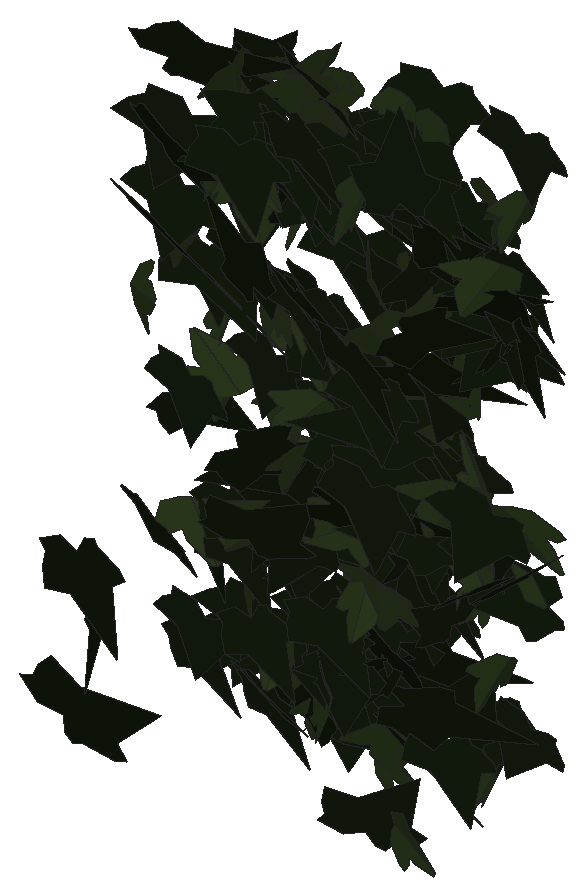
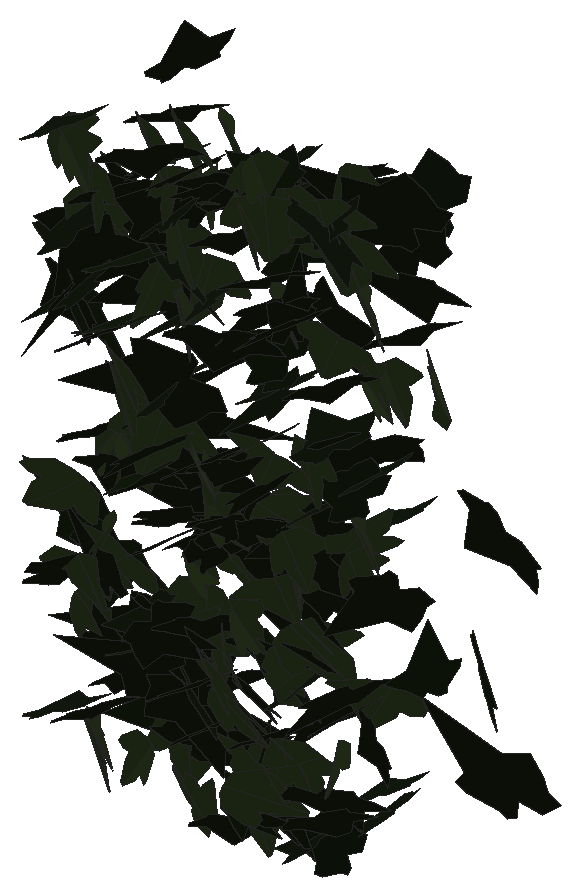
# SketchUp Ruby script. Lengths in millimetres.
U = 1.mm
M = Sketchup.active_model
def pt(a) = Geom::Point3d.new(a.map { |v| v * U })
def face(e, loops, mat)
  f = e.add_face(loops[0].map { |a| pt(a) })
  loops[1..].each { |l| e.add_face(l.map { |a| pt(a) }).erase! }
  f.material = f.back_material = mat if mat
  f
end
# faces: each face lists its corners as indices into pts; further lists are holes
def faces(e, pts, list, mat = nil) = list.each { |f| face(e, (f[0].is_a?(Array) ? f : [f]).map { |l| l.map { |i| pts[i] } }, mat) }
# xy, xz, yz: faces in a plane at the given z, y or x. An outline is a flat list of corners, or four numbers for a rectangle; further outlines are holes
def ring(l) = l.size == 4 ? [[l[0], l[1]], [l[2], l[1]], [l[2], l[3]], [l[0], l[3]]] : l.each_slice(2).to_a
def flat(e, list, mat, &to3) = list.each { |f| face(e, (f[0].is_a?(Array) ? f : [f]).map { |l| ring(l).map { |u, v| to3.(u, v) } }, mat) }
def xy(e, z, list, mat = nil) = flat(e, list, mat) { |x, y| [x, y, z] }
def xz(e, y, list, mat = nil) = flat(e, list, mat) { |x, z| [x, y, z] }
def yz(e, x, list, mat = nil) = flat(e, list, mat) { |y, z| [x, y, z] }
def lines(e, pts, list) = list.each { |a, b| e.add_line(pt(pts[a]), pt(pts[b])) }
# prism: a flat outline (further loops are holes) pulled along v
def prism(e, loops, v, mat = nil)
  f = face(e, loops, mat); d = Geom::Vector3d.new(v.map { |x| x * U })
  f.pushpull(f.normal.samedirection?(d) ? d.length : -d.length)
end
def box(e, o, s, mat = nil) = prism(e, [[o, [o[0] + s[0], o[1], o[2]], [o[0] + s[0], o[1] + s[1], o[2]], [o[0], o[1] + s[1], o[2]]]], [0, 0, s[2]], mat)
def at(x, y, z, deg = 0) = Geom::Transformation.translation(pt([x, y, z])) * Geom::Transformation.rotation(ORIGIN, Z_AXIS, deg.degrees)
def axes(o, x, y, z) = Geom::Transformation.new([*x, 0, *y, 0, *z, 0, *pt(o).to_a, 1])
def part(name) = M.definitions.add(name)
# library, detail: a bought-in or finely detailed component or shape, given as its bounding box
def library(name, o, s) = part(name).tap { |d| box(d.entities, o, s) }
def detail(e, o, s) = box(e.add_group.entities, o, s)
def put(e, d, t, mat = nil) = e.add_instance(d, t).tap { |i| i.material = mat if mat }
def group(e, t, mat = nil) = e.add_group.tap { |g| g.transformation = t; g.material = mat if mat }.entities
root = M.entities
M.materials.add("efeu1").color = [18, 25, 13]
M.materials.add("efeu2").color = [43, 57, 29]
c1 = part("ivyleaf_9")
p = [[39.1,54.8,31.7],[34.5,51.8,30.2],[-5.3,25.2,17.3],[-17.9,28.3,20.9],[-21.6,21.7,17],[-20.2,4.3,5.3],
  [-22.9,-0.3,2.5],[-17.1,-4,-0.6],[-2,-2.1,-1.2],[-0.7,-15.4,-10.1],[16.6,-22.3,-16.7],[21.1,-15.1,-12.5],
  [32.7,-10.7,-11],[46.1,-1.8,-6.6],[30.8,11.2,3.8]]
faces(c1.entities,p,[[0,1,2,3,4,5,6,7,8,9,10,11,12,13,14]],"efeu1")
c2 = part("ivyleaf_10")
p = [[0,12.8,-0.8],[-1.5,51.3,-10.9],[-4.9,51,-11.6],[-13.6,26.5,-7.3],[-13.2,15.9,-4.6],[-21.1,19.3,-7.2],
  [-29.5,16.3,-8.3],[-29.2,8.3,-6.2],[-19.7,-9.8,0.5],[-7.6,-13,4],[1,-12.2,5.8],[-0.4,51.1,-11.1],
  [-1.5,51.1,-10.9],[1,-12.4,5.9],[16.9,-12.4,3.5],[35.1,9.1,-5.1],[35,12.9,-6.1],[20.5,16.4,-4.9],
  [15.8,15,-3.8],[15.3,27.6,-7.1],[12.8,31.3,-7.8]]
faces(c2.entities,p,[[0,1,2,3,4,5,6,7,8,9,10],[11,12,0,13,14,15,16,17,18,19,20]],"efeu2")
put(root,c1,axes([4063.2,733.8,2968.8],[-0.0376,-0.17228,-1.13576],[-0.13622,1.13391,-0.17075],[2.18206,0.06782,-0.03023]))
put(root,c1,axes([4055.8,686.5,2823.3],[1.5513,-0.70151,-0.67063],[0.96409,-0.43949,1.07541],[-1.57548,-0.95968,-0.00226]))
put(root,c1,axes([4064.7,770.6,3133.3],[-0.07341,-1.05593,0.33534],[0.00836,-0.33568,-1.05651],[2.10853,-0.03543,0.01586]))
put(root,c1,axes([4039.1,548.3,2628],[-0.17639,0.13273,1.43159],[1.7479,-1.09826,0.16129],[2.10526,0.92296,-0.01396]))
put(root,c2,axes([4084,770.9,3056],[1.04005,-0.97402,0.24753],[0.21534,-0.22034,-1.11681],[1.90052,0.55799,-0.00892]))
put(root,c1,axes([4066.9,765.7,2785.8],[-0.57531,0.08526,-1.02674],[1.87322,-0.29236,-0.31405],[-0.57954,-1.02961,0.00416]))
put(root,c1,axes([4093.4,699.6,3351.9],[-1.90869,-0.57528,-0.28926],[0.46815,0.15249,-1.15613],[1.13254,-1.03257,-0.00959]))
put(root,c1,axes([4080.8,559.1,2788],[-1.15251,0.38599,-1.26243],[2.05887,-0.65093,-0.71794],[-1.43996,-1.23965,-0.0161]))
put(root,c2,axes([4096.2,739.7,3231],[0.60383,-0.99417,0.40773],[0.17674,-0.39817,-1.04313],[2.03739,0.32919,-0.03035]))
put(root,c2,axes([4103.2,692.9,3216.8],[-0.05357,-1.12054,0.09049],[0.02713,-0.09087,-1.12077],[2.13938,-0.02691,0.01648]))
put(root,c2,axes([4080.5,728.4,2825.7],[1.80422,0.56567,0.28702],[0.45808,0.15674,-1.10388],[-1.11695,0.97801,0.01091]))
put(root,c1,axes([4097,683.1,3269.7],[-0.81375,-1.09553,0.2771],[-0.1636,-0.26388,-1.17591],[2.14444,-0.43585,0.01544]))
put(root,c1,axes([4079.5,718.6,2670],[0.7911,-1.03663,-0.23213],[-0.16867,0.21457,-1.11686],[2.01473,0.425,-0.00235]))
put(root,c2,axes([4080.7,628,3159],[0.3126,-0.42355,-1.17811],[0.73038,-1.11397,0.454],[-2.26797,-0.41712,-0.01618]))
put(root,c1,axes([4092.3,728.3,2690.3],[-0.54384,-0.962,0.52983],[0.06228,-0.55469,-0.98948],[2.08927,-0.23387,0.16741]))
put(root,c2,axes([4104,758.4,2997.4],[-0.27143,-1.03123,0.33808],[0.28146,-0.35627,-1.02434],[2.04614,-0.08779,0.18575]))
put(root,c1,axes([4089.7,744.9,3159.3],[-0.50804,-1.01056,-0.71541],[0.35516,0.69065,-1.04522],[2.32956,-0.32568,0.00333]))
put(root,c2,axes([4121.9,734.9,3008.2],[0.77762,1.07105,0.31506],[-0.32067,-0.27249,1.14486],[2.10045,-0.43812,0.05815]))
put(root,c1,axes([4080.9,770.3,3102.2],[0.96558,-0.86425,0.57784],[0.61724,-0.47932,-1.00165],[1.87988,0.60129,0.03208]))
put(root,c1,axes([4103.7,689.3,3023.2],[-0.28326,-1.04741,0.50626],[0.0019,-0.5105,-1.05589],[2.21408,-0.13356,0.06568]))
put(root,c2,axes([4132.2,737.6,3396.3],[-2.16895,-0.0376,0.07781],[-0.13713,-0.15481,-1.13008],[0.09082,-1.13175,0.15199]))
put(root,c1,axes([4075.9,695.7,3426.5],[0.48012,-0.09617,1.25178],[2.3233,-0.2795,-0.26749],[0.55821,1.24599,0.03662]))
put(root,c1,axes([4102.7,766.8,2838.7],[0.44567,-1.05433,-0.74965],[-0.12292,0.75136,-1.0769],[2.45905,0.22864,0.08203]))
put(root,c2,axes([4126.8,756.3,2744],[0.82972,-0.6078,-0.72659],[0.17893,0.82366,-0.63259],[1.79398,0.19896,0.39914]))
put(root,c1,axes([4137.5,778.4,2696.3],[-1.66468,-0.6183,-0.07224],[0.11368,0.04065,-1.07114],[1.17928,-0.87671,0.00128]))
put(root,c1,axes([4153.8,752.9,3420.1],[0.08478,0.9438,0.64907],[-0.50152,0.64059,-0.91338],[-2.12156,-0.11371,0.24185]))
put(root,c1,axes([4123.8,785.4,3238.9],[-0.65034,-1.10482,0.04804],[-0.04197,-0.04346,-1.15642],[2.10425,-0.34232,-0.00822]))
put(root,c1,axes([4136.9,786,2669],[-1.10183,-0.84086,0.1464],[-0.20736,-0.10265,-1.02041],[1.6111,-0.58827,-0.03121]))
put(root,c1,axes([4115.6,753.5,2798],[0.33532,-1.10949,-0.16604],[-0.05444,0.16358,-1.12339],[2.1344,0.17848,-0.00257]))
put(root,c2,axes([4137.4,699.6,3310],[0.97597,-1.06387,0.03588],[0.01726,-0.03545,-1.18099],[2.02583,0.51284,-0.00722]))
put(root,c1,axes([4107.7,638.6,3349.5],[0.086,-0.46985,1.26714],[0.91479,-1.17936,-0.45444],[2.4039,0.46561,0.1276]))
put(root,c2,axes([4147.8,726.4,3397.1],[0.79933,-1.10899,0.09128],[0.06289,-0.08509,-1.18585],[2.11683,0.42129,0.00077]))
put(root,c1,axes([4122.4,772,3153.9],[-0.13685,-1.03136,0.75937],[0.46641,-0.75759,-1.00574],[2.3925,0.0887,0.2395]))
put(root,c2,axes([4165.5,740.5,3428.7],[-1.23255,-0.9441,0.09396],[-0.11242,-0.07342,-1.14485],[1.80219,-0.65027,-0.00715]))
put(root,c1,axes([4120.9,756,2616.5],[0.97697,-0.63278,0.63099],[0.70112,-0.51313,-0.81428],[1.5495,0.63115,-0.0294]))
put(root,c1,axes([4126.4,458.7,2902.9],[-1.02872,-0.11963,-1.31812],[2.51895,-0.04442,-0.53871],[0.00785,-1.42395,0.12754]))
put(root,c2,axes([4166.7,683.2,3448.6],[-0.27581,-1.12045,-0.49738],[0.24984,0.48378,-1.12806],[2.31969,-0.18533,0.06236]))
put(root,c2,axes([4146.5,735.2,3264],[2.06754,-0.06274,0.33696],[0.64867,0.07925,-1.08406],[0.06902,1.13464,0.09435]))
put(root,c1,axes([4142.8,736.9,3426.8],[1.39004,-0.87128,-0.24651],[-0.13994,0.2586,-1.13184],[1.71762,0.72618,0.10729]))
put(root,c2,axes([4196.1,733.8,2858.6],[-1.04434,-0.88,0.71355],[-0.73332,-0.60063,-1.03704],[2.02769,-0.67046,-0.00754]))
put(root,c2,axes([4178,748.8,3115.7],[1.47628,-0.66922,-0.42703],[-0.16127,0.52383,-0.97484],[1.50225,0.71389,0.315]))
put(root,c1,axes([4168.2,759.3,3042.9],[-0.46422,-0.97099,0.50201],[-0.09726,-0.50367,-0.99902],[2.0781,-0.24048,0.06539]))
put(root,c2,axes([4190.4,768.4,2999.6],[-0.51307,-1.04797,0.25565],[0.04854,-0.26963,-1.07839],[2.05241,-0.2556,0.08941]))
put(root,c1,axes([4163.5,749.8,2617.7],[0.65941,-1.05732,0.04467],[0.02539,-0.04263,-1.11264],[2.01392,0.34673,-0.0006]))
put(root,c2,axes([4195,740.5,2691.7],[1.11846,0.84094,-0.38065],[-0.38381,-0.32338,-1.02576],[-1.71436,0.62103,-0.01869]))
put(root,c2,axes([4211.6,757.3,2808.7],[-0.53133,-0.24398,-1.07687],[-0.77106,-1.01065,0.33401],[-1.95487,0.46494,0.16095]))
put(root,c1,axes([4229.3,642.6,3213.2],[0.03014,-0.13978,1.28616],[-0.63687,1.24204,0.1391],[-2.37843,-0.33435,-0.02095]))
put(root,c1,axes([4179.6,772.6,3297.9],[0.58629,-1.0062,-0.49226],[0.01513,0.51248,-1.04257],[2.13183,0.27308,0.14278]))
put(root,c2,axes([4215.7,733.6,2967.4],[0.46874,-0.95429,-0.66969],[-0.25051,0.65733,-0.98509],[2.20461,0.27759,0.03045]))
put(root,c1,axes([4194.8,688.8,2740.6],[0.25993,-1.03082,-0.47157],[-0.1751,0.46334,-1.03946],[2.15028,0.16234,-0.02764]))
put(root,c1,axes([4194.1,747.9,2801.2],[0.26781,-1.01076,0.2547],[0.02641,-0.25517,-1.0203],[1.98364,0.13986,-0.0208]))
put(root,c2,axes([4213.9,761.5,2936.6],[1.33131,0.82364,-0.35405],[-0.50455,-0.23895,-1.07966],[-1.62994,0.74671,0.04503]))
put(root,c1,axes([4211.2,738.8,3263.6],[0.41262,0.63503,0.99661],[-1.08999,-0.82983,0.65335],[1.9673,-0.59297,0.15297]))
put(root,c1,axes([4219.6,720,2898.2],[-1.98469,0.24053,-0.72523],[1.35006,-0.15119,-1.07015],[-0.54036,-1.26118,-0.01002]))
put(root,c1,axes([4169.3,518.9,3338.8],[1.63551,-1.02214,0.66736],[0.7842,-0.52536,-1.33523],[2.18691,0.95281,-0.0203]))
put(root,c1,axes([4246.2,665.8,3407.3],[-2.01004,-0.45578,0.43483],[-0.76096,-0.17091,-1.15029],[0.92642,-1.12929,-0.00141]))
put(root,c1,axes([4256.3,714.5,2950.4],[0.02781,-0.01696,-1.27934],[-1.4668,-1.02137,0.00473],[-1.94369,0.77053,-0.02188]))
put(root,c1,axes([4200.7,663.2,2977],[0.17879,0.19429,-1.26731],[-0.15454,1.26906,0.18854],[2.43524,0.06627,0.10501]))
put(root,c2,axes([4227.6,767.2,3424.6],[-1.80513,-0.68999,0.0723],[0.0172,-0.13474,-1.16733],[1.32026,-0.94163,0.11406]))
put(root,c2,axes([4232.5,726.9,2696.3],[-1.66169,-0.55762,0.13382],[-0.19637,-0.08703,-1.03583],[1.07359,-0.879,0.01767]))
put(root,c2,axes([4230,737.8,3425],[-1.17,-0.98924,-0.02006],[0.02942,0.01401,-1.16468],[1.88288,-0.61492,0.00574]))
put(root,c2,axes([4243.1,789.2,2666.6],[-0.31222,-0.42953,1.0688],[-0.74455,-0.99464,-0.45977],[2.06195,-0.42419,-0.00418]))
put(root,c2,axes([4187.9,667.2,3353.5],[1.42353,-0.10302,0.86127],[1.62715,-0.1045,-0.75498],[0.2788,1.13593,0.00866]))
put(root,c1,axes([4261.4,719.4,2650.4],[0.19101,0.10696,-1.20825],[-2.29195,0.15384,-0.08641],[0.27619,1.20261,0.11852]))
put(root,c2,axes([4240.3,738.8,3012],[-0.67676,-0.66207,0.84033],[-0.21575,-0.85723,-0.72336],[2.0246,-0.31266,0.20381]))
put(root,c1,axes([4256.2,728.9,2830],[-1.01019,0.94881,-0.14514],[0.13472,-0.12671,-1.08718],[-1.8218,-0.53549,0.00009]))
put(root,c1,axes([4233.7,746.5,2842.2],[-1.52416,-0.56478,-0.39797],[0.63872,0.21455,-0.97982],[1.14939,-0.86815,0.01676]))
put(root,c1,axes([4218.6,776,3071.5],[0.26785,-1.08394,-0.35961],[-0.15113,0.35216,-1.09258],[2.16826,0.15845,-0.03173]))
put(root,c1,axes([4211.5,664.3,2865.5],[-0.91298,-0.1477,1.03329],[1.92257,-0.352,0.41866],[0.50015,1.08347,0.27687]))
put(root,c1,axes([4235.6,766.8,2730.8],[-0.81684,-0.85852,0.41648],[-0.21116,-0.40867,-0.95676],[1.80373,-0.43663,0.0766]))
put(root,c2,axes([4240.1,725.3,3280.5],[0.91907,-1.0045,0.19161],[0.15523,-0.17339,-1.11455],[1.94003,0.48974,-0.00159]))
put(root,c2,axes([4246.7,752.7,3461.9],[-0.17986,-1.17257,0.14511],[0.01943,-0.14638,-1.17617],[2.24857,-0.09253,0.02177]))
put(root,c1,axes([4222.1,743.5,3291.5],[0.40376,-0.83368,-0.79645],[-0.0522,0.80594,-0.85092],[2.19372,0.17262,0.12634]))
put(root,c1,axes([4225.7,777.1,3125],[0.01219,-1.15086,0.10669],[0.02355,-0.10662,-1.15082],[2.19959,0.00752,0.01173]))
put(root,c2,axes([4223.9,755.5,3093.8],[2.0494,-0.16577,0.40576],[0.76537,-0.05449,-1.08948],[0.33184,1.14944,0.00687]))
put(root,c1,axes([4253.4,714.1,2866.4],[-1.94468,0.00735,-0.47474],[0.90306,-0.02459,-1.02164],[-0.0324,-1.12643,0.01921]))
put(root,c1,axes([4227.1,730.5,3172.1],[1.47111,-0.68624,-0.53505],[-0.56535,0.46457,-1.02499],[1.55663,0.81727,0.13338]))
put(root,c2,axes([4255.7,755.3,2637.3],[-0.35167,-1.22293,0.12241],[-0.00071,-0.12373,-1.23668],[2.3391,-0.1839,0.01803]))
put(root,c1,axes([4235.2,613.4,3398.7],[-0.43152,-1.19319,-0.1831],[0.05445,0.18094,-1.21453],[2.29681,-0.22846,-0.00561]))
put(root,c2,axes([4256.8,772.2,3412.4],[1.0182,-1.03638,-0.20639],[-0.08709,0.2084,-1.16506],[2.00928,0.53421,0.05409]))
put(root,c2,axes([4258.3,771.3,2879.3],[0.16209,-1.01726,0.47014],[0.17797,-0.4634,-1.01962],[2.12538,0.11638,0.04952]))
put(root,c1,axes([4267.9,718.9,2704.5],[0.67268,-0.02431,-0.98557],[-1.57698,0.55999,-0.31097],[1.01667,0.88469,0.16975]))
put(root,c1,axes([4267.2,777.4,2652],[-0.98887,0.44648,-0.79608],[0.85806,-0.67094,-0.67055],[-1.51041,-0.67347,0.14026]))
put(root,c1,axes([4250.9,745.7,3315.9],[-0.77389,-1.0623,0.14187],[0.10768,-0.17281,-1.13176],[2.03687,-0.39447,0.11374]))
put(root,c1,axes([4241.9,724.3,3165.8],[-0.1396,-1.08728,0.2572],[0.21766,-0.26371,-1.08217],[2.11525,-0.04462,0.12833]))
put(root,c2,axes([4267,687.3,2987.1],[-0.11857,-1.19015,0.11543],[0.02693,-0.11631,-1.19161],[2.27556,-0.06064,0.02012]))
put(root,c1,axes([4235,739.7,3440.6],[0.46896,-0.86973,0.69875],[0.60117,-0.63192,-0.89794],[2.03643,0.38683,0.10417]))
put(root,c1,axes([4256.3,774.3,3007.7],[-0.9981,-0.92448,-0.39502],[0.43043,0.32563,-1.06233],[1.86431,-0.57012,0.03378]))
put(root,c1,axes([4259.1,780.5,2623.1],[-0.8878,-0.9233,-0.21395],[0.22109,0.18096,-1.03422],[1.79018,-0.48024,0.02163]))
put(root,c1,axes([4231.8,687.2,3323.5],[0.3995,-0.86177,0.88202],[0.82821,-0.78537,-0.87091],[2.19589,0.453,0.16801]))
put(root,c2,axes([4244.3,764,2689.7],[1.88644,-0.35344,0.57322],[1.01577,-0.20974,-1.0522],[0.7816,1.12564,-0.01607]))
put(root,c2,axes([4305.9,750.2,2748.5],[-0.42466,0.31031,0.98176],[-1.86084,0.25103,-0.30156],[-0.61425,-0.975,0.23482]))
put(root,c1,axes([4254.2,770.1,3008.1],[0.15289,-0.81349,-0.76492],[0.20511,0.76896,-0.80648],[2.11525,-0.01576,0.13349]))
put(root,c1,axes([4266.5,774,3382.7],[-0.6259,-1.10495,-0.04858],[0.02014,0.04754,-1.15284],[2.10487,-0.32902,-0.00342]))
put(root,c1,axes([4252.9,687.5,3401.1],[0.44117,-1.16401,0.1185],[0.05641,-0.11492,-1.18685],[2.22608,0.2336,0.00659]))
put(root,c2,axes([4291,694.2,2671.5],[0.82687,-0.91011,-0.76698],[-0.38138,0.74889,-1.00216],[2.23284,0.46495,0.11286]))
put(root,c2,axes([4279.5,714.5,3428.3],[-0.82873,-0.94744,-0.49277],[0.4694,0.42855,-1.04192],[1.97753,-0.49877,0.04081]))
put(root,c1,axes([4268.6,667.3,3393.4],[-0.17249,-1.14355,-0.11002],[-0.02181,0.11126,-1.14696],[2.18635,-0.08911,-0.02012]))
put(root,c1,axes([4268.9,765,3078],[-0.35831,-0.9964,-0.41796],[0.26952,0.39785,-1.01223],[2.0387,-0.22772,0.06036]))
put(root,c1,axes([4295.5,741.2,2780.2],[-1.77743,0.13526,-0.46488],[0.84083,-0.1751,-0.93849],[-0.37694,-1.02843,0.09865]))
put(root,c1,axes([4315.4,733.2,2752.8],[-1.60526,0.63927,-0.03384],[0.04785,-0.02285,-1.05833],[-1.21742,-0.84382,0.00302]))
put(root,c2,axes([4297,763,3002.7],[-0.05013,-0.95141,0.54361],[-0.02503,-0.54345,-0.95178],[2.0853,-0.02939,0.00164]))
put(root,c1,axes([4272.3,660.9,3419.6],[0.75304,-1.07385,-0.1602],[-0.04301,0.16232,-1.14391],[2.06593,0.3948,0.03458]))
put(root,c1,axes([4260.3,689.3,3185.6],[0.89518,-1.01293,0.6329],[0.52857,-0.56881,-1.11676],[2.21088,0.54612,0.01073]))
put(root,c2,axes([4300.4,776.3,2803.2],[1.34924,-0.7746,-0.0278],[-0.03338,0.02163,-1.05004],[1.4748,0.70915,0.00166]))
put(root,c1,axes([4294.3,766.8,3237.2],[-1.23484,-0.85152,-0.45532],[0.51845,0.36487,-1.07053],[1.7631,-0.70368,-0.00411]))
put(root,c2,axes([4286.4,762.3,2819],[0.84868,-0.5792,0.75887],[0.96948,-0.56401,-0.7298],[1.53662,0.67574,0.04132]))
put(root,c1,axes([4284.4,707.5,2774.5],[0.06898,-1.08694,-0.38663],[0.17408,0.38831,-1.08309],[2.18873,0.00337,0.09833]))
put(root,c2,axes([4325.1,700.7,2906.2],[1.57109,-0.44156,-0.64322],[-1.10336,0.27952,-0.93591],[0.99371,1.00849,-0.02223]))
put(root,c1,axes([4315,770.7,2943.2],[0.09758,0.06212,1.16836],[-1.35858,-0.92493,0.0805],[1.76429,-0.71568,-0.00263]))
put(root,c1,axes([4299.3,785,2984.3],[-0.16774,-1.09101,-0.08498],[0.02618,0.08414,-1.09454],[2.08253,-0.08894,0.00691]))
put(root,c2,axes([4294.6,790.6,3051.3],[-0.07594,-0.23287,-1.08262],[0.72149,-1.02074,0.20559],[-1.98022,-0.36297,0.11642]))
put(root,c1,axes([4308.4,711.5,2714.5],[-1.39712,-0.39739,-0.63975],[1.30419,0.01816,-0.7976],[0.59461,-0.97357,0.24625]))
put(root,c2,axes([4342.2,734.6,2814.5],[-1.8238,0.06982,0.44465],[-0.83984,0.06024,-0.96048],[-0.1687,-1.05469,-0.02542]))
put(root,c2,axes([4323.9,750.9,3028.6],[-0.42262,0.56884,-0.97487],[-0.09959,-0.99768,-0.57023],[-2.14582,-0.06573,0.21847]))
put(root,c1,axes([4317.9,768.1,2855],[-0.55826,-1.01734,-0.37749],[0.21614,0.36011,-1.05875],[2.05385,-0.31442,0.00881]))
put(root,c1,axes([4317.8,763.5,3063.1],[-0.22688,-1.19443,0.09383],[0.00222,-0.09441,-1.20032],[2.28025,-0.11875,0.0105]))
put(root,c1,axes([4373.3,711.5,2649],[-0.08153,0.23918,1.108],[-2.14494,0.10964,-0.06724],[-0.23081,-1.1034,0.23349]))
put(root,c1,axes([4318.9,700.7,3400.8],[-0.49564,-1.07272,-0.67278],[0.48018,0.62913,-1.10079],[2.36159,-0.35306,0.08262]))
put(root,c1,axes([4333.1,751.3,2699.3],[-0.45212,-0.97421,0.30432],[-0.14545,-0.2946,-1.00275],[1.93703,-0.24951,-0.00426]))
put(root,c1,axes([4336.6,778.7,2766.7],[-0.6177,-1.02406,0.36522],[-0.08091,-0.3689,-1.07216],[2.06765,-0.32037,0.06715]))
put(root,c2,axes([4344.2,748.8,2913.9],[0.414,-0.74025,0.81435],[0.44611,-0.77989,-0.77155],[2.04644,0.31976,0.00345]))
put(root,c1,axes([4365,730.5,2730.3],[0.25472,1.10095,-0.43754],[-0.1058,-0.434,-1.10905],[-2.25225,0.1449,0.00262]))
put(root,c2,axes([4350.4,697.8,2825.7],[0.72833,0.90143,-0.42788],[-0.39394,-0.37659,-0.97849],[-1.85776,0.43326,0.03974]))
put(root,c1,axes([4337.8,687.9,3006.8],[-0.34511,-1.13237,0.18259],[0.00748,-0.18547,-1.14632],[2.18294,-0.17838,0.03279]))
put(root,c2,axes([4362.3,748.3,3334.7],[-0.27275,-1.12142,-0.0833],[0.0126,0.08313,-1.13053],[2.14012,-0.14341,-0.00396]))
put(root,c1,axes([4367.7,724.3,2730],[-1.51612,0.56117,-0.67503],[0.98861,-0.43348,-0.97337],[-1.34678,-0.94993,0.0454]))
put(root,c2,axes([4329.7,747.5,2589.6],[-0.54902,0.16868,1.14152],[1.84275,-0.6047,0.33404],[1.19467,1.01025,0.00935]))
put(root,c1,axes([4372.7,787.3,2842.5],[-0.29128,0.31302,-1.12692],[0.50656,-1.09739,-0.34097],[-2.16755,-0.29852,0.07175]))
put(root,c1,axes([4341.9,702.4,3384.4],[0.0256,-1.01618,-0.58211],[0.18774,0.58106,-1.01208],[2.22092,-0.0374,0.09226]))
put(root,c1,axes([4401.3,740.4,2815.3],[-1.81372,0.20387,-0.65346],[-1.23063,0.0995,0.97404],[0.42755,1.15121,0.03153]))
put(root,c1,axes([4384.2,714.3,2731.6],[0.72937,-0.84721,0.88138],[-0.75242,0.78816,0.9295],[-2.20172,-0.55001,-0.02568]))
put(root,c2,axes([4375,694.5,2838.4],[-1.87432,0.37039,0.21185],[-0.40349,0.03772,-1.05147],[-0.70476,-1.00665,0.03855]))
put(root,c2,axes([4374,735.5,3233.4],[0.57461,-1.02699,-0.35884],[-0.03732,0.36721,-1.06743],[2.07012,0.29169,0.08036]))
put(root,c1,axes([4409.4,701.4,3056.1],[-1.41495,-0.22338,0.9482],[-1.73859,-0.25443,-0.7762],[0.64396,-1.17775,-0.01216]))
put(root,c1,axes([4352.2,707.3,3236.3],[1.26402,-1.04697,-0.59352],[-0.32224,0.58987,-1.23],[2.26772,0.6674,0.15605]))
put(root,c1,axes([4360.1,739.4,3417.1],[0.29534,-1.10249,-0.27068],[-0.01528,0.27212,-1.11297],[2.16051,0.15263,0.02913]))
put(root,c1,axes([4335.3,663.5,2951.5],[1.01923,0.54877,-1.05958],[1.38844,0.76849,0.76673],[1.79714,-0.90495,0.00857]))
put(root,c2,axes([4393,703.5,2660],[-1.42136,-0.98188,-0.02551],[0.03112,0.01961,-1.23363],[1.86909,-0.747,0.00114]))
put(root,c2,axes([4381.2,722.1,3456.2],[1.54187,-0.83197,0.13658],[0.19799,-0.08932,-1.16119],[1.59234,0.81671,0.01214]))
put(root,c1,axes([4388.6,787.1,3453.1],[-0.91746,-1.03443,-0.13023],[0.089,0.12188,-1.1412],[1.98227,-0.48424,-0.00904]))
put(root,c2,axes([4396.4,711.6,3378.2],[-0.83541,-0.96935,-0.44434],[0.33334,0.40845,-1.06408],[2.0019,-0.47253,-0.00825]))
put(root,c1,axes([4383.8,672.1,3118.2],[-0.32639,-1.15961,0.09107],[-0.03838,-0.08908,-1.17221],[2.21344,-0.17254,-0.0069]))
put(root,c1,axes([4387.3,681,3010.3],[-1.03125,-0.95578,-0.49638],[0.39841,0.4516,-1.09807],[2.01063,-0.5797,-0.03701]))
put(root,c1,axes([4390.1,777.3,2798.6],[-0.70844,-0.982,0.234],[0.25421,-0.29512,-1.02601],[1.90437,-0.32591,0.22401]))
put(root,c1,axes([4379.8,775,3064.7],[0.43123,-1.04979,-0.45449],[-0.02988,0.46042,-1.07132],[2.17696,0.21427,0.07532]))
put(root,c2,axes([4403,738.6,3072.3],[-1.90253,-0.67534,-0.28068],[0.41558,0.17807,-1.20614],[1.32841,-1.02292,-0.02465]))
put(root,c2,axes([4404.8,610.7,3396.9],[1.12216,-1.08793,0.02339],[0.01971,-0.02099,-1.23743],[2.07093,0.58971,-0.00089]))
put(root,c1,axes([4401.5,741.5,3331.9],[-0.71923,-0.39798,1.02082],[-0.32697,-1.04495,-0.47099],[2.05946,-0.30489,0.28173]))
put(root,c1,axes([4439.3,707.8,2921],[-1.2282,-0.05727,0.86038],[-1.37933,-0.54624,-0.57996],[0.88918,-0.92646,0.28876]))
put(root,c2,axes([4411.8,633.1,3221.7],[-0.81445,-0.97958,-0.5903],[0.41184,0.54954,-1.0688],[2.13736,-0.47916,-0.01899]))
put(root,c1,axes([4405.1,751.6,2915.8],[-0.35414,-1.05331,0.25953],[-0.05253,-0.25864,-1.06948],[2.06395,-0.18731,0.01731]))
put(root,c1,axes([4443.2,694.9,3276.3],[-1.52866,0.90095,-0.27324],[0.35346,-0.20049,-1.20699],[-1.7566,-0.82438,-0.00508]))
put(root,c1,axes([4396.5,760.3,2831.9],[0.87884,-0.97188,0.05083],[0.04295,-0.04555,-1.076],[1.85172,0.46232,0.00083]))
put(root,c1,axes([4386.8,713.7,3125.4],[0.30765,0.40591,-1.21053],[1.00392,1.08996,0.43591],[2.21288,-0.55092,-0.02947]))
put(root,c2,axes([4428.4,727.7,3438.1],[1.35022,-0.86339,-0.28129],[-0.17761,0.28575,-1.11244],[1.71906,0.70766,0.106]))
put(root,c1,axes([4406.2,767.5,3014],[0.08319,-1.08023,0.24664],[0.11036,-0.24427,-1.0801],[2.10592,0.05547,0.04686]))
put(root,c2,axes([4445.8,591.4,3313.2],[-0.78245,0.4522,0.99052],[-1.17045,0.77729,-0.61011],[-1.71013,-0.7389,-0.03562]))
put(root,c2,axes([4422.3,747.4,2639.9],[-1.17723,0.8704,-0.15565],[0.17324,-0.12627,-1.0678],[-1.67388,-0.62521,-0.00104]))
put(root,c1,axes([4387.9,734.8,3335.1],[0.69214,-0.56307,0.97952],[1.25674,-0.72904,-0.66425],[1.74479,0.74848,0.08988]))
put(root,c2,axes([4431.3,779.2,3158.2],[1.42134,-0.83631,0.03138],[0.03263,-0.02676,-1.12121],[1.59245,0.74699,-0.00503]))
put(root,c1,axes([4420.3,753.4,3083.9],[-0.32972,-0.7848,0.82455],[-0.06178,-0.8303,-0.79709],[2.16559,-0.14318,0.1028]))
put(root,c1,axes([4418.2,615.2,2583.5],[-1.079,-0.08051,0.91684],[1.74966,0.00165,0.56862],[-0.08326,1.07797,0.06761]))
put(root,c2,axes([4431.1,705.6,3237.5],[-0.27778,-0.98591,-0.71835],[0.61185,0.66681,-0.98049],[2.23955,-0.30446,0.17877]))
put(root,c1,axes([4436.5,690.1,3444.1],[-1.05843,-0.98352,0.2666],[-0.06927,-0.28436,-1.12494],[1.93815,-0.54726,0.10538]))
put(root,c1,axes([4418.8,698.1,3394.8],[0.489,-1.07445,-0.4585],[0.01417,0.47096,-1.09947],[2.22326,0.23332,0.10785]))
put(root,c1,axes([4403.3,730.9,2745.9],[1.13088,0.26436,-0.83644],[0.95142,0.72812,0.58525],[1.3719,-0.72287,0.28361]))
put(root,c1,axes([4404.8,684,2672.5],[1.67153,-0.96416,0.25234],[0.3044,-0.19563,-1.30414],[1.87221,0.89262,-0.01325]))
put(root,c2,axes([4452.8,750.8,3118.5],[1.38932,-0.68407,-0.49113],[-0.3142,0.52111,-0.97121],[1.57162,0.7089,0.24]))
put(root,c1,axes([4446.6,767.1,3275.2],[-1.06222,-0.7736,0.61929],[-0.12212,-0.68105,-0.90858],[1.88201,-0.48082,0.29057]))
put(root,c1,axes([4414.1,707,3295.9],[-0.16966,0.04422,1.22627],[1.31172,-1.01542,0.08671],[1.93215,0.69324,0.0488]))
put(root,c1,axes([4481.9,683.6,2840.2],[-0.70626,0.9234,0.4039],[-0.3489,0.36138,-0.99464],[-1.88619,-0.41261,0.03275]))
put(root,c1,axes([4443.2,745.9,3006.3],[-1.04789,-0.74533,-0.55036],[0.73777,0.39616,-0.92432],[1.60157,-0.67016,0.0657]))
put(root,c1,axes([4455.7,773.4,3193.3],[-1.08529,-0.7939,0.63016],[-0.12674,-0.69213,-0.93224],[1.92491,-0.49319,0.29391]))
put(root,c1,axes([4441.1,657.5,3213.8],[0.18501,0.40459,-1.15688],[-0.28366,1.1558,0.39168],[2.31522,0.10928,0.14044]))
put(root,c2,axes([4430.8,768.1,2898],[1.83189,-0.19997,0.66872],[1.25669,-0.1083,-0.98281],[0.43053,1.16701,0.02338]))
put(root,c2,axes([4461.4,761.4,2924.6],[-0.45186,1.04211,-0.02396],[0.00949,-0.02344,-1.06881],[-1.98384,-0.23747,0.00035]))
put(root,c2,axes([4482.1,697.9,3002],[-1.36934,-0.90514,0.4233],[-0.3118,-0.4077,-1.15025],[1.87599,-0.72845,0.1178]))
put(root,c1,axes([4446.4,780.7,2868.8],[-0.11772,0.3458,1.07145],[0.54594,-1.03281,0.34989],[2.07203,0.29177,-0.03132]))
put(root,c1,axes([4460.2,570,3055.9],[-0.33968,-1.25088,0.38794],[0.0086,-0.39211,-1.26226],[2.49253,-0.16912,0.05723]))
put(root,c2,axes([4470.1,729.4,2995.8],[-0.22513,0.29675,-1.12846],[-0.0239,-1.13451,-0.29702],[-2.22058,-0.01788,0.11761]))
put(root,c1,axes([4472.1,742.9,3353.3],[-0.95304,-1.11948,0.18316],[-0.10309,-0.17639,-1.22617],[2.15647,-0.50318,0.02233]))
put(root,c2,axes([4473.1,750.9,2850.1],[-0.68535,-0.16195,1.05103],[0.66889,-1.06543,-0.04376],[1.91021,0.31497,0.39242]))
put(root,c1,axes([4472.1,778.6,2692.1],[-0.47167,-1.04448,0.09816],[0.00244,-0.10116,-1.0732],[1.99662,-0.24662,0.0245]))
put(root,c1,axes([4488.8,709.3,2871.5],[0.47491,1.00718,0.30349],[0.14054,0.29437,-1.03763],[-1.99706,0.26023,-0.00085]))
put(root,c2,axes([4496.9,721.5,2997.6],[-0.33468,1.04846,-0.50782],[-0.36291,0.48074,1.05859],[2.18727,0.24019,0.09794]))
put(root,c1,axes([4492.1,581.5,3440],[-1.13702,-0.67037,1.00603],[1.29404,0.74154,0.8979],[-1.90243,0.90506,0.00949]))
put(root,c1,axes([4490.3,772.1,3164.3],[-0.89825,-0.81281,0.70187],[-0.44344,-0.6709,-0.93362],[1.99517,-0.51505,0.10849]))
put(root,c2,axes([4489.7,770.8,2872.5],[2.0334,-0.01307,-0.20658],[-0.38923,0.10109,-1.0641],[0.06084,1.08349,0.09679]))
put(root,c2,axes([4493.2,743,3363.9],[1.20529,-0.81491,-0.47969],[0.02308,0.58428,-0.97658],[1.79953,0.53831,0.33381]))
put(root,c1,axes([4489.1,698.4,2706.8],[-1.49507,0.63276,0.59494],[0.64604,-0.51471,0.99563],[1.52151,0.84032,0.16185]))
put(root,c2,axes([4500.4,739.5,2633.5],[0.83163,-1.09032,-0.27127],[-0.1289,0.26497,-1.17411],[2.13447,0.44081,0.03479]))
put(root,c1,axes([4465.4,522.2,3260.1],[0.67652,-1.21612,0.46408],[0.27046,-0.44194,-1.26695],[2.46251,0.38264,0.01166]))
put(root,c1,axes([4456.1,645.1,2740.7],[0.81566,0.21806,-1.12222],[1.06856,1.00384,0.40947],[1.89528,-0.65981,0.2521]))
put(root,c2,axes([4500,737.6,2638],[0.91693,-0.93781,0.23175],[0.15611,-0.21832,-1.054],[1.83189,0.48801,-0.02618]))
put(root,c2,axes([4469.6,609.1,2597],[0.05415,-0.08076,1.0831],[1.8033,-0.52776,-0.06424],[1.0104,0.94624,0.05661]))
put(root,c1,axes([4487.3,674.9,2691.8],[-0.22564,-1.14911,-0.19067],[0.04398,0.1893,-1.1552],[2.21644,-0.12074,0.00351]))
put(root,c1,axes([4523.6,734.3,3194.6],[-1.13493,0.87273,-0.40941],[0.49665,-0.3173,-1.05646],[-1.76617,-0.65004,-0.03399]))
put(root,c1,axes([4491.4,754.8,3232.4],[1.33225,-0.81131,-0.51883],[-0.40894,0.49366,-1.06186],[1.78661,0.71798,0.14383]))
put(root,c1,axes([4542.8,778.1,2844],[-1.02532,-0.19896,0.96869],[-1.45871,-0.61306,-0.55217],[1.18932,-0.92345,0.15787]))
put(root,c1,axes([4505.5,699.6,3262.7],[1.65442,0.85438,0.20416],[0.28509,0.13884,-1.21885],[-1.64735,0.88207,-0.0059]))
put(root,c2,axes([4532.2,699.6,3304.7],[-1.12622,-0.8195,0.54675],[-0.17569,-0.58888,-0.98255],[1.86669,-0.54985,0.2374]))
put(root,c2,axes([4527.2,720.4,2785.3],[-0.21389,-0.95158,0.57292],[0.19612,-0.58229,-0.94693],[2.10483,-0.04244,0.14645]))
put(root,c1,axes([4520.3,780.8,2674],[-0.85303,-0.8113,0.54928],[0.06077,-0.6158,-0.8835],[1.86367,-0.35126,0.28022]))
put(root,c1,axes([4514.1,780.8,3439.7],[-0.33805,-1.06405,0.36521],[0.16476,-0.38156,-1.0696],[2.13471,-0.13905,0.14039]))
put(root,c2,axes([4534.4,735.7,3385.1],[0.1198,-1.17056,0.18926],[0.04759,-0.18818,-1.17216],[2.25623,0.06612,0.01467]))
put(root,c1,axes([4529.4,746.5,3199.6],[0.78266,-0.47929,-0.98265],[-1.0442,0.81762,-0.62841],[1.7998,0.68279,0.06272]))
put(root,c1,axes([4537.3,689.9,2995.7],[-1.05896,-1.02095,0.4111],[-0.23321,-0.40033,-1.16003],[2.08166,-0.56422,0.07918]))
put(root,c2,axes([4521.7,755.2,2958.9],[-1.77072,0.27639,-0.58135],[1.02917,-0.21868,-0.9694],[-0.66458,-1.07507,0.04773]))
put(root,c1,axes([4513.5,753.9,3291.5],[0.55349,-1.10386,0.3311],[0.22789,-0.31068,-1.14098],[2.18147,0.31253,0.03519]))
put(root,c1,axes([4523.6,706.3,2883.6],[0.60294,1.1083,0.15053],[-0.11207,-0.13971,1.15255],[2.12573,-0.32172,0.01807]))
put(root,c1,axes([4522.2,748.2,3203.2],[-0.62338,0.05392,-1.11872],[2.10879,-0.15453,-0.33186],[-0.31114,-1.15539,-0.00782]))
put(root,c2,axes([4554.9,724.6,3391.5],[-0.19438,-1.01703,0.53635],[0.26097,-0.54539,-1.00807],[2.17267,-0.02548,0.16907]))
